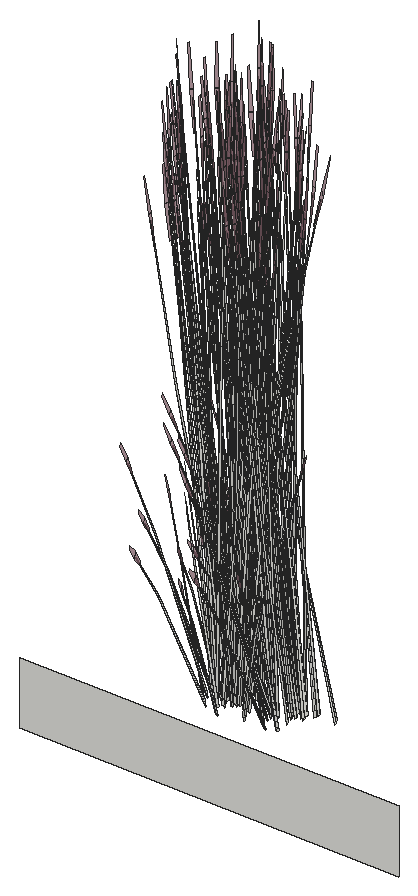
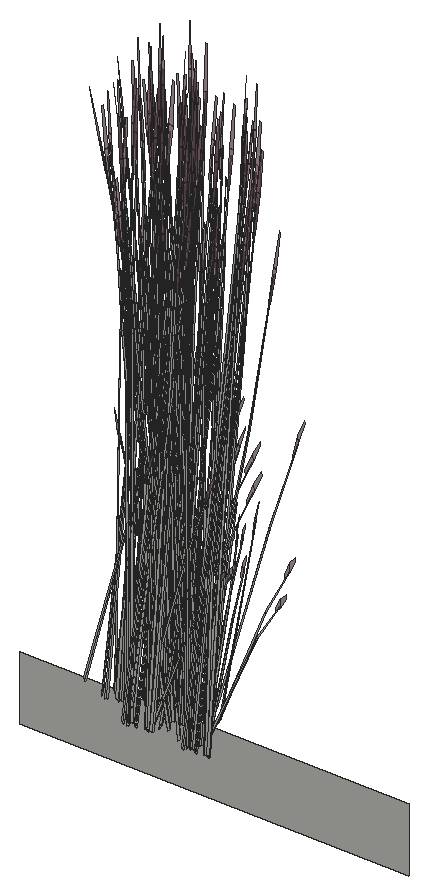
# SketchUp Ruby script. Lengths in inches.
U = 1.inch
M = Sketchup.active_model
def pt(a) = Geom::Point3d.new(a.map { |v| v * U })
def face(e, loops, mat)
  f = e.add_face(loops[0].map { |a| pt(a) })
  loops[1..].each { |l| e.add_face(l.map { |a| pt(a) }).erase! }
  f.material = f.back_material = mat if mat
  f
end
# faces: each face lists its corners as indices into pts; further lists are holes
def faces(e, pts, list, mat = nil) = list.each { |f| face(e, (f[0].is_a?(Array) ? f : [f]).map { |l| l.map { |i| pts[i] } }, mat) }
# xy, xz, yz: faces in a plane at the given z, y or x. An outline is a flat list of corners, or four numbers for a rectangle; further outlines are holes
def ring(l) = l.size == 4 ? [[l[0], l[1]], [l[2], l[1]], [l[2], l[3]], [l[0], l[3]]] : l.each_slice(2).to_a
def flat(e, list, mat, &to3) = list.each { |f| face(e, (f[0].is_a?(Array) ? f : [f]).map { |l| ring(l).map { |u, v| to3.(u, v) } }, mat) }
def xy(e, z, list, mat = nil) = flat(e, list, mat) { |x, y| [x, y, z] }
def xz(e, y, list, mat = nil) = flat(e, list, mat) { |x, z| [x, y, z] }
def yz(e, x, list, mat = nil) = flat(e, list, mat) { |y, z| [x, y, z] }
def lines(e, pts, list) = list.each { |a, b| e.add_line(pt(pts[a]), pt(pts[b])) }
# prism: a flat outline (further loops are holes) pulled along v
def prism(e, loops, v, mat = nil)
  f = face(e, loops, mat); d = Geom::Vector3d.new(v.map { |x| x * U })
  f.pushpull(f.normal.samedirection?(d) ? d.length : -d.length)
end
def box(e, o, s, mat = nil) = prism(e, [[o, [o[0] + s[0], o[1], o[2]], [o[0] + s[0], o[1] + s[1], o[2]], [o[0], o[1] + s[1], o[2]]]], [0, 0, s[2]], mat)
def at(x, y, z, deg = 0) = Geom::Transformation.translation(pt([x, y, z])) * Geom::Transformation.rotation(ORIGIN, Z_AXIS, deg.degrees)
def axes(o, x, y, z) = Geom::Transformation.new([*x, 0, *y, 0, *z, 0, *pt(o).to_a, 1])
def part(name) = M.definitions.add(name)
# library, detail: a bought-in or finely detailed component or shape, given as its bounding box
def library(name, o, s) = part(name).tap { |d| box(d.entities, o, s) }
def detail(e, o, s) = box(e.add_group.entities, o, s)
def put(e, d, t, mat = nil) = e.add_instance(d, t).tap { |i| i.material = mat if mat }
def group(e, t, mat = nil) = e.add_group.tap { |g| g.transformation = t; g.material = mat if mat }.entities
root = M.entities
M.materials.add("LightPink_Translucent").color = [144, 107, 117]
M.materials["LightPink_Translucent"].alpha = 0.75
c1 = part("blade")
p = [[2.15,0.21,22],[0,0.17,0],[0.09,0.45,0],[2.18,0.31,22],[2.29,0.31,22],[0.38,0.45,0],
  [2.48,0.24,33],[2.49,0.24,33],[2.48,0.22,33]]
faces(c1.entities,p,[[0,1,2,3],[4,5,2,3],[6,3,4,7],[8,0,3,6]])
c2 = part("seeds")
p = [[0.3,-0.1,1.38],[-0.01,-0.03,1.59],[-0.01,-0.03,0.03],[0.14,-0.07,-0.07],[0.29,-0.03,3],[0.15,0.01,3.11]]
faces(c2.entities,p,[[0,1,2,3],[1,0,4,5]],"LightPink_Translucent")
c3 = part("blade with seeds")
put(c3.entities,c1,at(0,0,0))
put(c3.entities,c2,axes([2.4,0.25,30.99],[1.5799,-0.05474,1.17369],[-0.12525,1.92788,0.29478],[-0.07173,-0.02425,1.56792]))
xz(root,14,[[310,42,346,48]])
put(root,c3,axes([329.52,14.96,50.29],[-0.14352,0.07909,1.26356],[-0.42983,-0.13843,-0.27174],[0.07968,-0.17216,0.54024]))
put(root,c3,axes([327.29,14.81,50.29],[-0.03058,0.12783,1.26356],[-0.44698,0.10701,-0.27174],[-0.10448,-0.16522,0.54024]))
put(root,c3,axes([332.95,14.81,50.29],[-0.03058,0.12783,1.26356],[-0.44698,0.10701,-0.27174],[-0.10448,-0.16522,0.54024]))
put(root,c3,axes([328.45,14.53,49.32],[-0.08469,0.01408,1.55816],[-0.46834,-0.15847,-0.23804],[0.00786,-0.13218,0.26541]))
put(root,c3,axes([326.93,15.01,49.32],[-0.04891,0.05148,1.55816],[-0.49427,0.11098,-0.23804],[-0.1194,-0.10096,0.26541]))
put(root,c3,axes([332.59,15.01,49.32],[-0.04891,0.05148,1.55816],[-0.49427,0.11098,-0.23804],[-0.1194,-0.10096,0.26541]))
put(root,c3,axes([327.75,16.42,49.85],[-0.20736,-0.4007,-0.61707],[0.59731,-0.14431,-0.16195],[-0.02292,-0.13569,1.36206]))
put(root,c3,axes([333.4,16.42,49.85],[-0.20736,-0.4007,-0.61707],[0.59731,-0.14431,-0.16195],[-0.02292,-0.13569,1.36206]))
put(root,c3,axes([330.52,15.2,49.32],[-0.07557,-0.03078,1.55816],[-0.19412,-0.34391,-0.23804],[0.13095,-0.09333,0.26541]))
put(root,c3,axes([327.67,15.27,50.1],[-0.31568,-0.39156,0],[0.52815,-0.21836,-0.456],[0.12029,-0.04973,1.44655]))
put(root,c3,axes([328.36,14.8,49.88],[-0.34892,0.22417,-0.0344],[-0.3197,-0.24551,-0.15595],[-0.02251,-0.06957,0.51438]))
put(root,c3,axes([334.01,14.8,49.88],[-0.34892,0.22417,-0.0344],[-0.3197,-0.24551,-0.15595],[-0.02251,-0.06957,0.51438]))
put(root,c3,axes([326.52,16.37,49.78],[0,-0.39075,-0.43871],[0.56491,0,0],[0,-0.089,1.3917]))
put(root,c3,axes([332.18,16.37,49.78],[0,-0.39075,-0.43871],[0.56491,0,0],[0,-0.089,1.3917]))
put(root,c3,axes([328.09,15.21,49.78],[0.47255,-0.19538,-0.43871],[0.28245,0.35034,0],[0.10763,-0.0445,1.3917]))
put(root,c3,axes([328.65,16.01,49.82],[0.34009,-0.2937,-0.55095],[0.42248,0.26632,-0.1446],[0.13628,-0.07327,1.21613]))
put(root,c3,axes([328.0625,16.53,49.95],[0.24498,-0.3521,-0.39531],[0.50902,0.16945,0.19025],[0,-0.08116,1.26923]))
put(root,c3,axes([328.29,16.35,50.36],[-0.05884,-0.44587,-0.25709],[0.6128,-0.02696,-0.44182],[0.10791,-0.05939,1.41118]))
put(root,c3,axes([326.77,16.375,49.79],[0.35245,-0.2438,-0.27372],[0.35245,0.2438,0.27372],[0,-0.07853,1.22797]))
put(root,c3,axes([332.42,16.375,49.79],[0.35245,-0.2438,-0.27372],[0.35245,0.2438,0.27372],[0,-0.07853,1.22797]))
put(root,c3,axes([326.625,15.21,49.88],[-0.14565,0.31907,-0.0344],[-0.44829,-0.09815,-0.15595],[-0.06806,-0.05219,0.51438]))
put(root,c3,axes([332.28,15.21,49.88],[-0.14565,0.31907,-0.0344],[-0.44829,-0.09815,-0.15595],[-0.06806,-0.05219,0.51438]))
put(root,c3,axes([328,16.82,50.36],[-0.56863,-0.18645,-0.25709],[0.2738,-0.39352,-0.44182],[-0.01787,-0.09662,1.41118]))
put(root,c3,axes([333.66,16.82,50.36],[-0.56863,-0.18645,-0.25709],[0.2738,-0.39352,-0.44182],[-0.01787,-0.09662,1.41118]))
put(root,c3,axes([326.38,16.66,50.1],[-0.63136,0,0],[0,-0.43672,-0.456],[0,-0.09947,1.44655]))
put(root,c3,axes([332.04,16.66,50.1],[-0.63136,0,0],[0,-0.43672,-0.456],[0,-0.09947,1.44655]))
put(root,c3,axes([332.15,15.88,50.29],[0.09858,0.10879,1.26356],[-0.22716,0.29571,-0.27174],[-0.23325,-0.07068,0.54024]))
put(root,c3,axes([328.2,15.37,49.79],[0.47106,0.09668,-0.27372],[-0.11861,0.34048,0.27372],[0.09497,-0.03926,1.22797]))
put(root,c3,axes([326.87,16.55,50.06],[-0.46965,0.32852,0.27176],[-0.46994,-0.32506,-0.32244],[-0.0164,-0.09329,1.45692]))
put(root,c3,axes([332.53,16.55,50.06],[-0.46965,0.32852,0.27176],[-0.46994,-0.32506,-0.32244],[-0.0164,-0.09329,1.45692]))
put(root,c3,axes([328.37,16.7,50.15],[0.56891,0.18939,0.21263],[-0.2738,0.39352,0.44182],[0,-0.09071,1.41855]))
put(root,c3,axes([330.09,18.21,50.29],[-0.03058,0.12783,1.26356],[-0.44698,0.10701,-0.27174],[-0.10448,-0.16522,0.54024]))
put(root,c3,axes([328.14,17.23,50.16],[0.13383,-0.46302,-0.20702],[0.63453,0.08071,0.45303],[-0.11087,-0.06394,1.38231]))
put(root,c3,axes([333.8,17.23,50.16],[0.13383,-0.46302,-0.20702],[0.63453,0.08071,0.45303],[-0.11087,-0.06394,1.38231]))
put(root,c3,axes([331.24,17.93,49.32],[-0.08469,0.01408,1.55816],[-0.46834,-0.15847,-0.23804],[0.00786,-0.13218,0.26541]))
put(root,c3,axes([326.49,18.66,50.29],[-0.14352,0.07909,1.26356],[-0.42983,-0.13843,-0.27174],[0.07968,-0.17216,0.54024]))
put(root,c3,axes([328.18,16.4375,50.4],[-0.54829,0.02412,0.39531],[-0.04958,-0.40041,-0.19025],[0.09816,-0.04058,1.26923]))
put(root,c3,axes([326.77,16.73,50.19],[0,0.39075,0.43871],[-0.56491,0,0],[0,-0.089,1.3917]))
put(root,c3,axes([332.42,16.73,50.19],[0,0.39075,0.43871],[-0.56491,0,0],[0,-0.089,1.3917]))
put(root,c3,axes([329.99,15.37,50.1],[0.31568,-0.39156,0],[0.52815,0.21836,-0.456],[0.12029,0.04973,1.44655]))
put(root,c3,axes([328.1,17.05,49.95],[-0.30332,-0.32798,-0.39531],[0.45944,-0.23096,0.19025],[-0.09816,-0.04058,1.26923]))
put(root,c3,axes([333.76,17.05,49.95],[-0.30332,-0.32798,-0.39531],[0.45944,-0.23096,0.19025],[-0.09816,-0.04058,1.26923]))
put(root,c3,axes([328.16,16.58,50.09],[0.21952,0.43694,0.40429],[-0.62724,0.15194,0.15865],[0.00767,-0.08029,1.40366]))
put(root,c3,axes([325.42,18.23,49.32],[-0.08469,0.01408,1.55816],[-0.46834,-0.15847,-0.23804],[0.00786,-0.13218,0.26541]))
put(root,c3,axes([328.05,16.93,50.4],[-0.24498,0.3521,0.39531],[-0.50902,-0.16945,-0.19025],[0,-0.08116,1.26923]))
put(root,c3,axes([328.95,16.62,49.95],[0,-0.45213,0],[0.63136,0,0],[0,0,1.58567]))
put(root,c3,axes([329.72,15.57,50.19],[-0.47255,-0.19538,0.43871],[0.28245,-0.35034,0],[0.10763,0.0445,1.3917]))
put(root,c3,axes([327.83,17.17,49.82],[-0.52523,-0.06406,-0.55095],[0.11084,-0.39517,-0.1446],[-0.15674,-0.04788,1.21613]))
put(root,c3,axes([333.48,17.17,49.82],[-0.52523,-0.06406,-0.55095],[0.11084,-0.39517,-0.1446],[-0.15674,-0.04788,1.21613]))
put(root,c3,axes([328.65,16.33,50.09],[-0.41865,0.35461,0.40429],[-0.49737,-0.31303,0.15865],[0.10093,-0.03539,1.40366]))
put(root,c3,axes([329.11,16.97,50.03],[-0.46965,-0.33633,-0.05417],[0.46994,-0.33653,0],[-0.0164,-0.01174,1.55135]))
put(root,c3,axes([327.93,15.75,50.1875],[-0.14586,0.38834,0.15589],[-0.53375,-0.1099,0.31002],[0.0922,-0.00189,1.41735]))
put(root,c3,axes([327.71,16.0625,49.41],[-0.49699,0.15644,1.13921],[-0.15819,-0.44887,0.44265],[0.30518,0.00747,1.29573]))
put(root,c3,axes([329.04,16.18,50.3125],[0.09741,-0.34873,0.12794],[0.4759,0.06053,-0.36534],[0.08661,0.03581,1.11991]))
put(root,c3,axes([328.22,17.01,50.09],[0.63817,0.08233,0.40429],[-0.12987,0.46497,0.15865],[-0.09326,-0.0449,1.40366]))
put(root,c3,axes([326.14,16.61,49.32],[0.0128,0.06158,1.55816],[-0.25814,0.3216,-0.23804],[-0.18336,-0.01621,0.26541]))
put(root,c3,axes([331.8,16.61,49.32],[0.0128,0.06158,1.55816],[-0.25814,0.3216,-0.23804],[-0.18336,-0.01621,0.26541]))
put(root,c3,axes([328.84,16.27,50.4],[-0.30332,-0.32798,0.39531],[0.45944,-0.23096,-0.19025],[0.09816,0.04058,1.26923]))
put(root,c3,axes([327.27,17.77,49.79],[-0.11861,-0.34048,-0.27372],[0.47106,-0.09668,0.27372],[-0.09497,-0.03926,1.22797]))
put(root,c3,axes([332.93,17.77,49.79],[-0.11861,-0.34048,-0.27372],[0.47106,-0.09668,0.27372],[-0.09497,-0.03926,1.22797]))
put(root,c3,axes([327.875,17.75,50.1875],[0.54257,-0.10371,0.15589],[0.13397,0.38597,0.31002],[-0.04839,-0.05624,1.41735]))
put(root,c3,axes([328.99,16.3,50.36],[0.50979,-0.25942,-0.25709],[0.339,0.36656,-0.44182],[0.12578,0.03723,1.41118]))
put(root,c3,axes([329.73,18.41,49.32],[-0.04891,0.05148,1.55816],[-0.49427,0.11098,-0.23804],[-0.1194,-0.10096,0.26541]))
put(root,c3,axes([327.14,17.92,49.78],[-0.47255,-0.19538,-0.43871],[0.28245,-0.35034,0],[-0.10763,-0.0445,1.3917]))
put(root,c3,axes([332.79,17.92,49.78],[-0.47255,-0.19538,-0.43871],[0.28245,-0.35034,0],[-0.10763,-0.0445,1.3917]))
put(root,c3,axes([330.54,19.82,49.85],[-0.20736,-0.4007,-0.61707],[0.59731,-0.14431,-0.16195],[-0.02292,-0.13569,1.36206]))
put(root,c3,axes([330.28,15.61,49.78],[0.47255,0.19538,-0.43871],[-0.28245,0.35034,0],[0.10763,0.0445,1.3917]))
put(root,c3,axes([329.38,16.72,49.95],[0.56491,0,0],[0,0.40454,0],[0,0,1.5764]))
put(root,c3,axes([328.42,17.23,50.36],[-0.50979,0.25942,-0.25709],[-0.339,-0.36656,-0.44182],[-0.12578,-0.03723,1.41118]))
put(root,c3,axes([334.08,17.23,50.36],[-0.50979,0.25942,-0.25709],[-0.339,-0.36656,-0.44182],[-0.12578,-0.03723,1.41118]))
put(root,c3,axes([329.54,15.77,50.1875],[-0.54257,0.10371,0.15589],[-0.13397,-0.38597,0.31002],[0.04839,0.05624,1.41735]))
put(root,c3,axes([330.15,15.75,49.79],[0.11861,0.34048,-0.27372],[-0.47106,0.09668,0.27372],[0.09497,0.03926,1.22797]))
put(root,c3,axes([324.73,20.13,49.85],[-0.20736,-0.4007,-0.61707],[0.59731,-0.14431,-0.16195],[-0.02292,-0.13569,1.36206]))
put(root,c3,axes([327.5,18.91,49.32],[-0.07557,-0.03078,1.55816],[-0.19412,-0.34391,-0.23804],[0.13095,-0.09333,0.26541]))
put(root,c3,axes([329.2,16.51,50.1],[-0.63817,-0.08233,0.43472],[0.12987,-0.46497,0.17059],[0.09326,0.0449,1.50931]))
put(root,c3,axes([328.69,17.66,49.95],[-0.16474,-0.33688,0],[0.47043,-0.11798,0],[0,0,1.36402]))
put(root,c3,axes([330.46,18.67,50.1],[-0.31568,-0.39156,0],[0.52815,-0.21836,-0.456],[0.12029,-0.04973,1.44655]))
put(root,c3,axes([328.375,17.34,50.3125],[-0.09741,0.34873,0.12794],[-0.4759,-0.06053,-0.36534],[-0.08661,-0.03581,1.11991]))
put(root,c3,axes([334.03,17.34,50.3125],[-0.09741,0.34873,0.12794],[-0.4759,-0.06053,-0.36534],[-0.08661,-0.03581,1.11991]))
put(root,c3,axes([331.15,18.2,49.88],[-0.34892,0.22417,-0.0344],[-0.3197,-0.24551,-0.15595],[-0.02251,-0.06957,0.51438]))
put(root,c3,axes([329.31,17.62,49.93],[0.53009,-0.13258,-0.16963],[0.18627,0.38191,0.00007],[0.05851,-0.01465,1.53656]))
put(root,c3,axes([329.49,17.77,50.1875],[0.14586,-0.38834,0.15589],[0.53375,0.1099,0.31002],[-0.0922,0.00189,1.41735]))
put(root,c3,axes([329.37,16.89,49.96],[0.35245,0.2524,0],[-0.35245,0.2524,0],[0,0,1.49564]))
put(root,c3,axes([330.32,16.78,50.1875],[-0.39671,-0.28463,0.15589],[0.39978,-0.27607,0.31002],[-0.04381,0.05813,1.41735]))
put(root,c3,axes([324.64,18.98,50.1],[-0.31568,-0.39156,0],[0.52815,-0.21836,-0.456],[0.12029,-0.04973,1.44655]))
put(root,c3,axes([328.57,17.82,49.94],[-0.50902,-0.17543,0],[0.24498,-0.36452,0],[0,0,1.43768]))
put(root,c3,axes([329,17.35,50.18],[-0.49304,-0.31451,-0.2226],[0.41487,-0.35316,0.48713],[-0.13277,0.03679,1.48635]))
put(root,c3,axes([334.65,17.35,50.18],[-0.49304,-0.31451,-0.2226],[0.41487,-0.35316,0.48713],[-0.13277,0.03679,1.48635]))
put(root,c3,axes([327.7,17.95,50.19],[0.47255,0.19538,0.43871],[-0.28245,0.35034,0],[-0.10763,-0.0445,1.3917]))
put(root,c3,axes([333.35,17.95,50.19],[0.47255,0.19538,0.43871],[-0.28245,0.35034,0],[-0.10763,-0.0445,1.3917]))
put(root,c3,axes([325.34,18.51,49.88],[-0.34892,0.22417,-0.0344],[-0.3197,-0.24551,-0.15595],[-0.02251,-0.06957,0.51438]))
put(root,c3,axes([329.32,19.77,49.78],[0,-0.39075,-0.43871],[0.56491,0,0],[0,-0.089,1.3917]))
put(root,c3,axes([329.36,16.6,50.4],[0.24498,-0.3521,0.39531],[0.50902,0.16945,-0.19025],[0,0.08116,1.26923]))
put(root,c3,axes([329.27,16.8,50.03],[0,0.45191,-0.04981],[-0.63136,0,0],[0,0.0142,1.58489]))
put(root,c3,axes([329.32,16.48,49.95],[0.30332,0.32798,-0.39531],[-0.45944,0.23096,0.19025],[0.09816,0.04058,1.26923]))
put(root,c3,axes([327.43,18.16,50.1],[-0.31568,0.39156,0],[-0.52815,-0.21836,-0.456],[-0.12029,-0.04973,1.44655]))
put(root,c3,axes([333.08,18.16,50.1],[-0.31568,0.39156,0],[-0.52815,-0.21836,-0.456],[-0.12029,-0.04973,1.44655]))
put(root,c3,axes([330.65,16.8,50.19],[0,-0.39075,0.43871],[0.56491,0,0],[0,0.089,1.3917]))
put(root,c3,axes([329.23,17.09,50.4],[0.54829,-0.02412,0.39531],[0.04958,0.40041,-0.19025],[-0.09816,0.04058,1.26923]))
put(root,c3,axes([329.58,16.68,50.3125],[0.47043,-0.11396,0.12794],[0.16474,0.32541,-0.36534],[0,0.07162,1.11991]))
put(root,c3,axes([323.5,20.08,49.78],[0,-0.39075,-0.43871],[0.56491,0,0],[0,-0.089,1.3917]))
put(root,c3,axes([325.07,18.92,49.78],[0.47255,-0.19538,-0.43871],[0.28245,0.35034,0],[0.10763,-0.0445,1.3917]))
put(root,c3,axes([327.88,19.59,50.29],[-0.18038,-0.01157,1.26356],[-0.18479,-0.31048,-0.27174],[0.22159,-0.08783,0.54024]))
put(root,c3,axes([328.75,17.28,49.95],[-0.54829,0.02412,-0.39531],[-0.04958,-0.40041,0.19025],[-0.09816,0.04058,1.26923]))
put(root,c3,axes([334.4,17.28,49.95],[-0.54829,0.02412,-0.39531],[-0.04958,-0.40041,0.19025],[-0.09816,0.04058,1.26923]))
put(root,c3,axes([330.86,19.93,49.95],[0.24498,-0.3521,-0.39531],[0.50902,0.16945,0.19025],[0,-0.08116,1.26923]))
put(root,c3,axes([325.63,19.72,49.82],[0.34009,-0.2937,-0.55095],[0.42248,0.26632,-0.1446],[0.13628,-0.07327,1.21613]))
put(root,c3,axes([331.08,19.75,50.36],[-0.05884,-0.44587,-0.25709],[0.6128,-0.02696,-0.44182],[0.10791,-0.05939,1.41118]))
put(root,c3,axes([329.5625,19.78,49.79],[0.35245,-0.2438,-0.27372],[0.35245,0.2438,0.27372],[0,-0.07853,1.22797]))
put(root,c3,axes([329.42,18.61,49.88],[-0.14565,0.31907,-0.0344],[-0.44829,-0.09815,-0.15595],[-0.06806,-0.05219,0.51438]))
put(root,c3,axes([330.8,20.22,50.36],[-0.56863,-0.18645,-0.25709],[0.2738,-0.39352,-0.44182],[-0.01787,-0.09662,1.41118]))
put(root,c3,axes([329.15,17.82,49.95],[0.50902,0.17543,0],[-0.24498,0.36452,0],[0,0,1.54589]))
put(root,c3,axes([329.18,20.06,50.1],[-0.63136,0,0],[0,-0.43672,-0.456],[0,-0.09947,1.44655]))
put(root,c3,axes([329.29,19.28,50.29],[0.09858,0.10879,1.26356],[-0.22716,0.29571,-0.27174],[-0.23325,-0.07068,0.54024]))
put(root,c3,axes([329.35,18.21,49.9375],[-0.31175,-0.39292,-0.04544],[0.52815,-0.21836,0.456],[-0.13015,0.03741,1.44584]))
put(root,c3,axes([335.01,18.21,49.9375],[-0.31175,-0.39292,-0.04544],[0.52815,-0.21836,0.456],[-0.13015,0.03741,1.44584]))
put(root,c3,axes([325.04,20.24,49.95],[0.24498,-0.3521,-0.39531],[0.50902,0.16945,0.19025],[0,-0.08116,1.26923]))
put(root,c3,axes([329.24,17.26,50.3125],[0.37303,0.23477,0.12794],[-0.31115,0.26487,-0.36534],[-0.08661,0.03581,1.11991]))
put(root,c3,axes([325.26,20.0625,50.36],[-0.05884,-0.44587,-0.25709],[0.6128,-0.02696,-0.44182],[0.10791,-0.05939,1.41118]))
put(root,c3,axes([323.75,20.09,49.79],[0.35245,-0.2438,-0.27372],[0.35245,0.2438,0.27372],[0,-0.07853,1.22797]))
put(root,c3,axes([324.98,20.53,50.36],[-0.56863,-0.18645,-0.25709],[0.2738,-0.39352,-0.44182],[-0.01787,-0.09662,1.41118]))
put(root,c3,axes([325.18,19.07,49.79],[0.47106,0.09668,-0.27372],[-0.11861,0.34048,0.27372],[0.09497,-0.03926,1.22797]))
put(root,c3,axes([329.64,17.98,50.19],[0.47255,-0.19538,0.43871],[0.28245,0.35034,0],[-0.10763,0.0445,1.3917]))
put(root,c3,axes([328.97,17.67,50.02],[0.21952,0.44891,-0.05313],[-0.62724,0.1573,0],[0.00767,0.01568,1.52132]))
put(root,c3,axes([329.21,18.16,49.79],[-0.47106,-0.09668,-0.27372],[0.11861,-0.34048,0.27372],[-0.09497,0.03926,1.22797]))
put(root,c3,axes([334.87,18.16,49.79],[-0.47106,-0.09668,-0.27372],[0.11861,-0.34048,0.27372],[-0.09497,0.03926,1.22797]))
put(root,c3,axes([329.67,19.95,50.06],[-0.46965,0.32852,0.27176],[-0.46994,-0.32506,-0.32244],[-0.0164,-0.09329,1.45692]))
put(root,c3,axes([331.47,17.47,50.29],[0.17547,0.03208,1.26356],[0.1131,0.32764,-0.27174],[-0.23835,0.06133,0.54024]))
put(root,c3,axes([337.07,17.47,50.29],[0.17547,0.03208,1.26356],[0.1131,0.32764,-0.27174],[-0.23835,0.06133,0.54024]))
put(root,c3,axes([331.03,16.86,50.1],[0.63136,0,0],[0,0.43672,-0.456],[0,0.09947,1.44655]))
put(root,c3,axes([330.78,17.09,49.94],[-0.63105,-0.00312,-0.04397],[0,-0.43672,0.44129],[-0.01983,0.09942,1.3992]))
put(root,c3,axes([329.42,16.71,50.36],[0.56863,0.18645,-0.25709],[-0.2738,0.39352,-0.44182],[0.01787,0.09662,1.41118]))
put(root,c3,axes([331.16,20.1,50.15],[0.56891,0.18939,0.21263],[-0.2738,0.39352,0.44182],[0,-0.09071,1.41855]))
put(root,c3,axes([330.94,20.63,50.16],[0.13383,-0.46302,-0.20702],[0.63453,0.08071,0.45303],[-0.11087,-0.06394,1.38231]))
put(root,c3,axes([330.65,17.15,49.79],[-0.35245,0.2438,-0.27372],[-0.35245,-0.2438,0.27372],[0,0.07853,1.22797]))
put(root,c3,axes([329.13,17.17,50.36],[0.05884,0.44587,-0.25709],[-0.6128,0.02696,-0.44182],[-0.10791,0.05939,1.41118]))
put(root,c3,axes([334.79,17.17,50.36],[0.05884,0.44587,-0.25709],[-0.6128,0.02696,-0.44182],[-0.10791,0.05939,1.41118]))
put(root,c3,axes([329.35,17,49.95],[-0.24498,0.3521,-0.39531],[-0.50902,-0.16945,0.19025],[0,0.08116,1.26923]))
put(root,c3,axes([323.85,20.26,50.06],[-0.46965,0.32852,0.27176],[-0.46994,-0.32506,-0.32244],[-0.0164,-0.09329,1.45692]))
put(root,c3,axes([330.98,19.84,50.4],[-0.54829,0.02412,0.39531],[-0.04958,-0.40041,-0.19025],[0.09816,-0.04058,1.26923]))
put(root,c3,axes([329.5625,20.13,50.19],[0,0.39075,0.43871],[-0.56491,0,0],[0,-0.089,1.3917]))
put(root,c3,axes([325.34,20.41,50.15],[0.56891,0.18939,0.21263],[-0.2738,0.39352,0.44182],[0,-0.09071,1.41855]))
put(root,c3,axes([325.125,20.94,50.16],[0.13383,-0.46302,-0.20702],[0.63453,0.08071,0.45303],[-0.11087,-0.06394,1.38231]))
put(root,c3,axes([330.9,20.45,49.95],[-0.30332,-0.32798,-0.39531],[0.45944,-0.23096,0.19025],[-0.09816,-0.04058,1.26923]))
put(root,c3,axes([330.96,19.98,50.09],[0.21952,0.43694,0.40429],[-0.62724,0.15194,0.15865],[0.00767,-0.08029,1.40366]))
put(root,c3,axes([328.76,17.51,49.82],[-0.34009,0.2937,-0.55095],[-0.42248,-0.26632,-0.1446],[-0.13628,0.07327,1.21613]))
put(root,c3,axes([334.42,17.51,49.82],[-0.34009,0.2937,-0.55095],[-0.42248,-0.26632,-0.1446],[-0.13628,0.07327,1.21613]))
